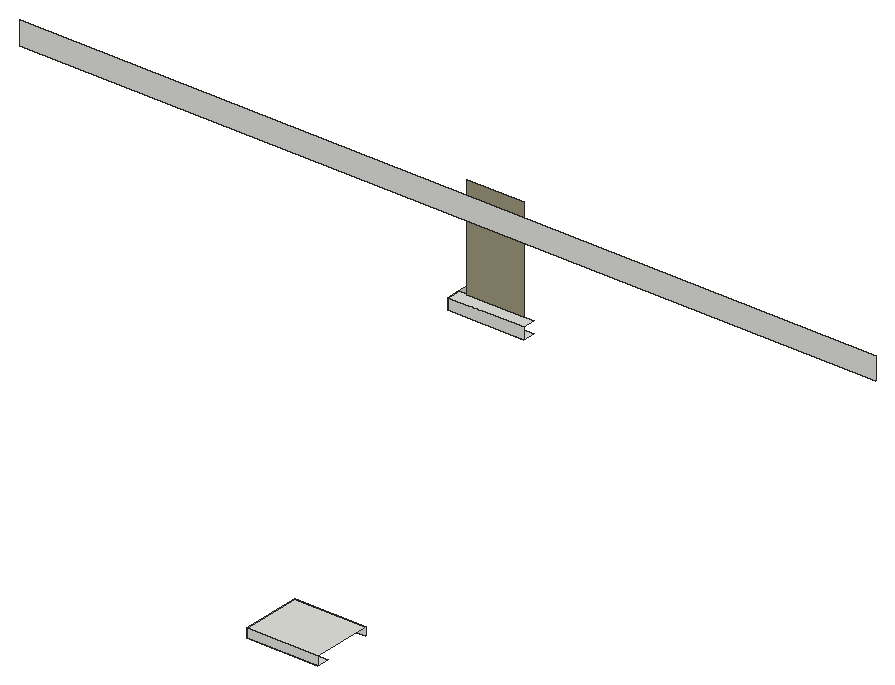
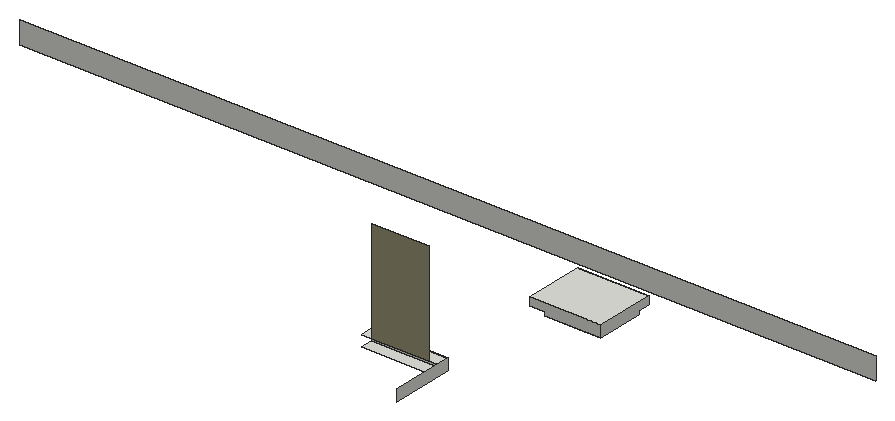
# SketchUp Ruby script. Lengths in inches.
U = 1.inch
M = Sketchup.active_model
def pt(a) = Geom::Point3d.new(a.map { |v| v * U })
def face(e, loops, mat)
  f = e.add_face(loops[0].map { |a| pt(a) })
  loops[1..].each { |l| e.add_face(l.map { |a| pt(a) }).erase! }
  f.material = f.back_material = mat if mat
  f
end
# faces: each face lists its corners as indices into pts; further lists are holes
def faces(e, pts, list, mat = nil) = list.each { |f| face(e, (f[0].is_a?(Array) ? f : [f]).map { |l| l.map { |i| pts[i] } }, mat) }
# xy, xz, yz: faces in a plane at the given z, y or x. An outline is a flat list of corners, or four numbers for a rectangle; further outlines are holes
def ring(l) = l.size == 4 ? [[l[0], l[1]], [l[2], l[1]], [l[2], l[3]], [l[0], l[3]]] : l.each_slice(2).to_a
def flat(e, list, mat, &to3) = list.each { |f| face(e, (f[0].is_a?(Array) ? f : [f]).map { |l| ring(l).map { |u, v| to3.(u, v) } }, mat) }
def xy(e, z, list, mat = nil) = flat(e, list, mat) { |x, y| [x, y, z] }
def xz(e, y, list, mat = nil) = flat(e, list, mat) { |x, z| [x, y, z] }
def yz(e, x, list, mat = nil) = flat(e, list, mat) { |y, z| [x, y, z] }
def lines(e, pts, list) = list.each { |a, b| e.add_line(pt(pts[a]), pt(pts[b])) }
# prism: a flat outline (further loops are holes) pulled along v
def prism(e, loops, v, mat = nil)
  f = face(e, loops, mat); d = Geom::Vector3d.new(v.map { |x| x * U })
  f.pushpull(f.normal.samedirection?(d) ? d.length : -d.length)
end
def box(e, o, s, mat = nil) = prism(e, [[o, [o[0] + s[0], o[1], o[2]], [o[0] + s[0], o[1] + s[1], o[2]], [o[0], o[1] + s[1], o[2]]]], [0, 0, s[2]], mat)
def at(x, y, z, deg = 0) = Geom::Transformation.translation(pt([x, y, z])) * Geom::Transformation.rotation(ORIGIN, Z_AXIS, deg.degrees)
def axes(o, x, y, z) = Geom::Transformation.new([*x, 0, *y, 0, *z, 0, *pt(o).to_a, 1])
def part(name) = M.definitions.add(name)
# library, detail: a bought-in or finely detailed component or shape, given as its bounding box
def library(name, o, s) = part(name).tap { |d| box(d.entities, o, s) }
def detail(e, o, s) = box(e.add_group.entities, o, s)
def put(e, d, t, mat = nil) = e.add_instance(d, t).tap { |i| i.material = mat if mat }
def group(e, t, mat = nil) = e.add_group.tap { |g| g.transformation = t; g.material = mat if mat }.entities
root = M.entities
M.materials.add("[Blinds Vertical Stripe Gray]").color = [160, 160, 160]
M.materials.add("[Stone Coursed Rough]").color = [155, 150, 122]
xy(root,57.8125,[[188.52,96.24,192.64,111],[192.64,96.24,206.19,111]])
xy(root,58.8125,[[188.52,92.49,210.69,96.24]])
xy(root,61.4375,[[188.52,92.49,210.69,111]])
xy(root,95.36,[[165.87,199.23,189.49,203.17]])
xy(root,98.875,[[165.87,199.23,189.49,203.17]])
xz(root,92.49,[[188.52,58.8125,210.69,61.4375]])
xz(root,96.24,[[188.52,57.8125,192.64,58.8125],[192.64,57.8125,206.19,58.8125]],"[Blinds Vertical Stripe Gray]")
xz(root,111,[[188.52,57.8125,188.52,61.4375,210.69,61.4375,210.69,58.8125,206.19,58.8125,206.19,57.8125]])
xz(root,187.36,[[41.9,130.875,308.53,137.875]])
xz(root,199.23,[[165.87,95.36,189.49,98.875]])
xz(root,203.17,[[168.55,98.875,186.24,130.875]],"[Stone Coursed Rough]")
yz(root,165.87,[[199.23,95.36,219.06,98.875]])
yz(root,188.52,[[96.24,57.8125,96.24,58.8125,92.49,58.8125,92.49,61.4375,111,61.4375,111,57.8125]])
